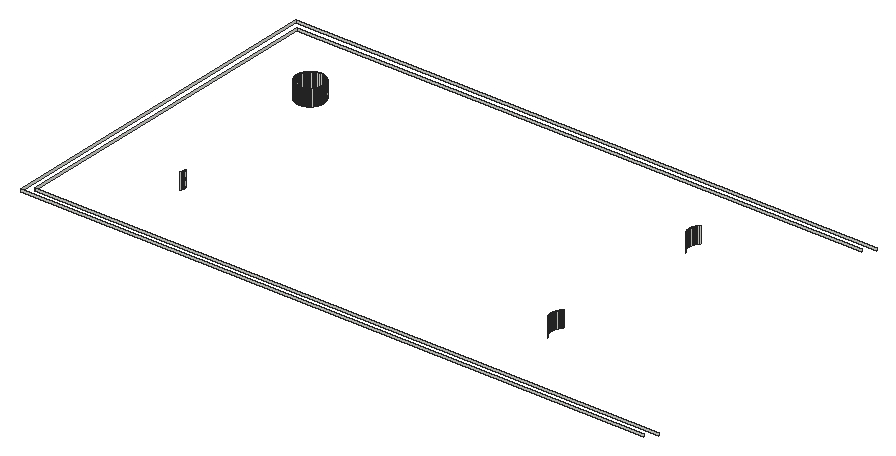
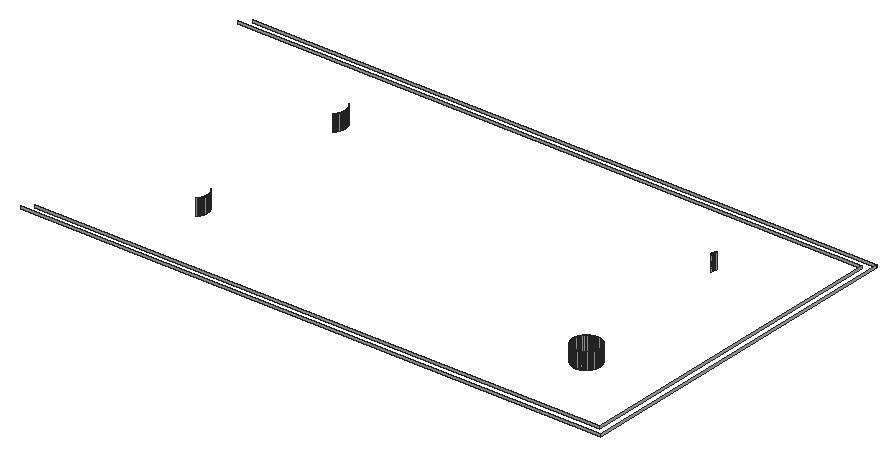
# SketchUp Ruby script. Lengths in inches.
U = 1.inch
M = Sketchup.active_model
def pt(a) = Geom::Point3d.new(a.map { |v| v * U })
def face(e, loops, mat)
  f = e.add_face(loops[0].map { |a| pt(a) })
  loops[1..].each { |l| e.add_face(l.map { |a| pt(a) }).erase! }
  f.material = f.back_material = mat if mat
  f
end
# faces: each face lists its corners as indices into pts; further lists are holes
def faces(e, pts, list, mat = nil) = list.each { |f| face(e, (f[0].is_a?(Array) ? f : [f]).map { |l| l.map { |i| pts[i] } }, mat) }
# xy, xz, yz: faces in a plane at the given z, y or x. An outline is a flat list of corners, or four numbers for a rectangle; further outlines are holes
def ring(l) = l.size == 4 ? [[l[0], l[1]], [l[2], l[1]], [l[2], l[3]], [l[0], l[3]]] : l.each_slice(2).to_a
def flat(e, list, mat, &to3) = list.each { |f| face(e, (f[0].is_a?(Array) ? f : [f]).map { |l| ring(l).map { |u, v| to3.(u, v) } }, mat) }
def xy(e, z, list, mat = nil) = flat(e, list, mat) { |x, y| [x, y, z] }
def xz(e, y, list, mat = nil) = flat(e, list, mat) { |x, z| [x, y, z] }
def yz(e, x, list, mat = nil) = flat(e, list, mat) { |y, z| [x, y, z] }
def lines(e, pts, list) = list.each { |a, b| e.add_line(pt(pts[a]), pt(pts[b])) }
# prism: a flat outline (further loops are holes) pulled along v
def prism(e, loops, v, mat = nil)
  f = face(e, loops, mat); d = Geom::Vector3d.new(v.map { |x| x * U })
  f.pushpull(f.normal.samedirection?(d) ? d.length : -d.length)
end
def box(e, o, s, mat = nil) = prism(e, [[o, [o[0] + s[0], o[1], o[2]], [o[0] + s[0], o[1] + s[1], o[2]], [o[0], o[1] + s[1], o[2]]]], [0, 0, s[2]], mat)
def at(x, y, z, deg = 0) = Geom::Transformation.translation(pt([x, y, z])) * Geom::Transformation.rotation(ORIGIN, Z_AXIS, deg.degrees)
def axes(o, x, y, z) = Geom::Transformation.new([*x, 0, *y, 0, *z, 0, *pt(o).to_a, 1])
def part(name) = M.definitions.add(name)
# library, detail: a bought-in or finely detailed component or shape, given as its bounding box
def library(name, o, s) = part(name).tap { |d| box(d.entities, o, s) }
def detail(e, o, s) = box(e.add_group.entities, o, s)
def put(e, d, t, mat = nil) = e.add_instance(d, t).tap { |i| i.material = mat if mat }
def group(e, t, mat = nil) = e.add_group.tap { |g| g.transformation = t; g.material = mat if mat }.entities
root = M.entities
xz(root,184,[[22,116,138,116.5]])
xz(root,185.5,[[23.5,116,139.5,116.5]])
xz(root,229.5,[[37.34,116,37.42,119],[37.42,116,37.5,119],[37.5,116,37.58,119],[37.58,116,37.66,119]])
xz(root,234.5,[[37.34,116,37.42,119],[37.42,116,37.5,119],[37.5,116,37.58,119],[37.58,116,37.66,119]])
xz(root,246.5,[[23.5,116,128.5,116.5]])
xz(root,248,[[22,116,130,116.5]])
yz(root,22,[[184,116,248,116.5]])
yz(root,23.5,[[185.5,116,246.5,116.5]])
yz(root,35,[[231.84,116,231.92,119],[231.92,116,232,119],[232,116,232.08,119],[232.08,116,232.16,119]])
yz(root,40,[[199.84,116,199.92,119],[199.92,116,200,119],[231.84,116,231.92,119],[231.92,116,232,119],[232,116,232.08,119],
  [232.08,116,232.16,119]])
yz(root,108,[[199.84,116,199.92,119],[199.92,116,200,119],[200,116,200.08,119],[200.08,116,200.16,119],[231.84,116,231.92,119],
  [231.92,116,232,119],[232,116,232.08,119],[232.08,116,232.16,119]])
p = [[108.73,198.23,116],[108.68,198.29,116],[108.68,198.29,119],[108.73,198.23,119],[108.79,198.18,116],[108.79,198.18,119],
  [108.625,198.35,116],[108.57,198.41,116],[108.57,198.41,119],[108.625,198.35,119],[108.52,198.47,116],[108.52,198.47,119],
  [108.48,198.53,116],[108.43,198.59,116],[108.43,198.59,119],[108.48,198.53,119],[108.39,198.66,116],[108.39,198.66,119],
  [108.35,198.73,116],[108.31,198.8,116],[108.31,198.8,119],[108.35,198.73,119],[108.27,198.87,116],[108.27,198.87,119],
  [39.79,199.01,116],[39.76,198.9375,116],[39.76,198.9375,119],[39.79,199.01,119],[108.24,198.9375,116],[108.21,199.01,116],
  [108.21,199.01,119],[108.24,198.9375,119],[39.82,199.08,116],[39.82,199.08,119],[108.18,199.08,116],[108.18,199.08,119],
  [39.85,199.15,116],[39.85,199.15,119],[108.15,199.15,116],[108.15,199.15,119],[39.88,199.23,116],[39.88,199.23,119],
  [39.9,199.3,116],[39.9,199.3,119],[108.12,199.23,116],[108.1,199.3,116],[108.1,199.3,119],[108.12,199.23,119],
  [39.92,199.38,116],[39.92,199.38,119],[108.08,199.38,116],[108.08,199.38,119],[39.94,199.45,116],[39.94,199.45,119],
  [108.06,199.45,116],[108.06,199.45,119],[39.96,199.53,116],[39.96,199.53,119],[39.97,199.61,116],[39.97,199.61,119],
  [108.04,199.53,116],[108.03,199.61,116],[108.03,199.61,119],[108.04,199.53,119],[39.98,199.6875,116],[39.98,199.6875,119],
  [108.02,199.6875,116],[108.02,199.6875,119],[39.99,199.76,116],[39.99,199.76,119],[108.01,199.76,116],[108.01,199.76,119],
  [40,199.84,116],[40,199.84,119],[108,199.84,116],[108,199.84,119],[108,200.16,116],[108.01,200.24,116],
  [108.01,200.24,119],[108,200.16,119],[108.02,200.3125,116],[108.02,200.3125,119],[108.03,200.39,116],[108.03,200.39,119],
  [108.04,200.47,116],[108.04,200.47,119],[108.06,200.55,116],[108.06,200.55,119],[108.08,200.62,116],[108.08,200.62,119],
  [108.1,200.7,116],[108.1,200.7,119],[108.12,200.77,116],[108.12,200.77,119],[108.15,200.85,116],[108.15,200.85,119],
  [108.18,200.92,116],[108.18,200.92,119],[108.21,200.99,116],[108.21,200.99,119],[108.24,201.0625,116],[108.24,201.0625,119],
  [108.27,201.13,116],[108.27,201.13,119],[108.31,201.2,116],[108.31,201.2,119],[108.35,201.27,116],[108.35,201.27,119],
  [108.39,201.34,116],[108.39,201.34,119],[108.43,201.41,116],[108.43,201.41,119],[108.48,201.47,116],[108.48,201.47,119],
  [108.52,201.53,116],[108.52,201.53,119],[108.57,201.59,116],[108.57,201.59,119],[108.625,201.65,116],[108.625,201.65,119],
  [108.68,201.71,116],[108.68,201.71,119],[108.73,201.77,116],[108.73,201.77,119],[108.79,201.82,116],[108.79,201.82,119],
  [37.03,229.54,116],[36.95,229.56,116],[36.95,229.56,119],[37.03,229.54,119],[37.11,229.53,116],[37.11,229.53,119],
  [37.1875,229.52,116],[37.1875,229.52,119],[37.26,229.51,116],[37.26,229.51,119],[37.34,229.5,116],[37.34,229.5,119],
  [37.74,229.51,116],[37.66,229.5,116],[37.66,229.5,119],[37.74,229.51,119],[37.8125,229.52,116],[37.8125,229.52,119],
  [37.89,229.53,116],[37.89,229.53,119],[37.97,229.54,116],[37.97,229.54,119],[38.05,229.56,116],[38.05,229.56,119],
  [36.65,229.65,116],[36.58,229.68,116],[36.58,229.68,119],[36.65,229.65,119],[36.73,229.62,116],[36.73,229.62,119],
  [36.8,229.6,116],[36.8,229.6,119],[36.88,229.58,116],[36.88,229.58,119],[38.12,229.58,116],[38.12,229.58,119],
  [38.2,229.6,116],[38.2,229.6,119],[38.27,229.62,116],[38.27,229.62,119],[38.35,229.65,116],[38.35,229.65,119],
  [38.42,229.68,116],[38.42,229.68,119],[36.4375,229.74,116],[36.37,229.77,116],[36.37,229.77,119],[36.4375,229.74,119],
  [36.51,229.71,116],[36.51,229.71,119],[38.49,229.71,116],[38.49,229.71,119],[38.5625,229.74,116],[38.5625,229.74,119],
  [38.63,229.77,116],[38.63,229.77,119],[36.23,229.85,116],[36.16,229.89,116],[36.16,229.89,119],[36.23,229.85,119],
  [36.3,229.81,116],[36.3,229.81,119],[38.7,229.81,116],[38.7,229.81,119],[38.77,229.85,116],[38.77,229.85,119],
  [38.84,229.89,116],[38.84,229.89,119],[36.09,229.93,116],[36.03,229.98,116],[36.03,229.98,119],[36.09,229.93,119],
  [38.91,229.93,116],[38.91,229.93,119],[38.97,229.98,116],[38.97,229.98,119],[35.97,230.02,116],[35.91,230.07,116],
  [35.91,230.07,119],[35.97,230.02,119],[39.03,230.02,116],[39.03,230.02,119],[39.09,230.07,116],[39.09,230.07,119],
  [35.85,230.125,116],[35.79,230.18,116],[35.79,230.18,119],[35.85,230.125,119],[39.15,230.125,116],[39.15,230.125,119],
  [39.21,230.18,116],[39.21,230.18,119],[35.73,230.23,116],[35.68,230.29,116],[35.68,230.29,119],[35.73,230.23,119],
  [39.27,230.23,116],[39.27,230.23,119],[39.32,230.29,116],[39.32,230.29,119],[108.73,230.23,116],[108.68,230.29,116],
  [108.68,230.29,119],[108.73,230.23,119],[108.79,230.18,116],[108.79,230.18,119],[35.625,230.35,116],[35.57,230.41,116],
  [35.57,230.41,119],[35.625,230.35,119],[39.375,230.35,116],[39.375,230.35,119],[39.43,230.41,116],[39.43,230.41,119],
  [108.625,230.35,116],[108.57,230.41,116],[108.57,230.41,119],[108.625,230.35,119],[35.52,230.47,116],[35.52,230.47,119],
  [39.48,230.47,116],[39.48,230.47,119],[108.52,230.47,116],[108.52,230.47,119],[35.48,230.53,116],[35.43,230.59,116],
  [35.43,230.59,119],[35.48,230.53,119],[39.52,230.53,116],[39.52,230.53,119],[39.57,230.59,116],[39.57,230.59,119],
  [108.48,230.53,116],[108.43,230.59,116],[108.43,230.59,119],[108.48,230.53,119],[35.39,230.66,116],[35.39,230.66,119],
  [39.61,230.66,116],[39.61,230.66,119],[108.39,230.66,116],[108.39,230.66,119],[35.35,230.73,116],[35.31,230.8,116],
  [35.31,230.8,119],[35.35,230.73,119],[39.65,230.73,116],[39.65,230.73,119],[39.69,230.8,116],[39.69,230.8,119],
  [108.35,230.73,116],[108.31,230.8,116],[108.31,230.8,119],[108.35,230.73,119],[35.27,230.87,116],[35.27,230.87,119],
  [39.73,230.87,116],[39.73,230.87,119],[108.27,230.87,116],[108.27,230.87,119],[35.24,230.9375,116],[35.21,231.01,116],
  [35.21,231.01,119],[35.24,230.9375,119],[39.76,230.9375,116],[39.76,230.9375,119],[39.79,231.01,116],[39.79,231.01,119],
  [108.24,230.9375,116],[108.21,231.01,116],[108.21,231.01,119],[108.24,230.9375,119],[35.18,231.08,116],[35.18,231.08,119],
  [39.82,231.08,116],[39.82,231.08,119],[108.18,231.08,116],[108.18,231.08,119],[35.15,231.15,116],[35.15,231.15,119],
  [39.85,231.15,116],[39.85,231.15,119],[108.15,231.15,116],[108.15,231.15,119],[35.12,231.23,116],[35.1,231.3,116],
  [35.1,231.3,119],[35.12,231.23,119],[39.88,231.23,116],[39.88,231.23,119],[39.9,231.3,116],[39.9,231.3,119],
  [108.12,231.23,116],[108.1,231.3,116],[108.1,231.3,119],[108.12,231.23,119],[35.08,231.38,116],[35.08,231.38,119],
  [39.92,231.38,116],[39.92,231.38,119],[108.08,231.38,116],[108.08,231.38,119],[35.06,231.45,116],[35.06,231.45,119],
  [39.94,231.45,116],[39.94,231.45,119],[108.06,231.45,116],[108.06,231.45,119],[35.04,231.53,116],[35.03,231.61,116],
  [35.03,231.61,119],[35.04,231.53,119],[39.96,231.53,116],[39.96,231.53,119],[39.97,231.61,116],[39.97,231.61,119],
  [108.04,231.53,116],[108.03,231.61,116],[108.03,231.61,119],[108.04,231.53,119],[35.02,231.6875,116],[35.02,231.6875,119],
  [39.98,231.6875,116],[39.98,231.6875,119],[108.02,231.6875,116],[108.02,231.6875,119],[35.01,231.76,116],[35.01,231.76,119],
  [39.99,231.76,116],[39.99,231.76,119],[108.01,231.76,116],[108.01,231.76,119],[35,231.84,116],[35,231.84,119],
  [40,231.84,116],[40,231.84,119],[108,231.84,116],[108,231.84,119],[35,232.16,116],[35.01,232.24,116],
  [35.01,232.24,119],[35,232.16,119],[35.02,232.3125,116],[35.02,232.3125,119],[39.98,232.3125,116],[39.99,232.24,116],
  [39.99,232.24,119],[39.98,232.3125,119],[40,232.16,116],[40,232.16,119],[108,232.16,116],[108.01,232.24,116],
  [108.01,232.24,119],[108,232.16,119],[108.02,232.3125,116],[108.02,232.3125,119],[35.03,232.39,116],[35.03,232.39,119],
  [39.97,232.39,116],[39.97,232.39,119],[108.03,232.39,116],[108.03,232.39,119],[35.04,232.47,116],[35.04,232.47,119],
  [39.96,232.47,116],[39.96,232.47,119],[108.04,232.47,116],[108.04,232.47,119],[35.06,232.55,116],[35.06,232.55,119],
  [35.08,232.62,116],[35.08,232.62,119],[39.92,232.62,116],[39.94,232.55,116],[39.94,232.55,119],[39.92,232.62,119],
  [108.06,232.55,116],[108.06,232.55,119],[108.08,232.62,116],[108.08,232.62,119],[35.1,232.7,116],[35.1,232.7,119],
  [39.9,232.7,116],[39.9,232.7,119],[108.1,232.7,116],[108.1,232.7,119],[35.12,232.77,116],[35.12,232.77,119],
  [39.88,232.77,116],[39.88,232.77,119],[108.12,232.77,116],[108.12,232.77,119],[35.15,232.85,116],[35.15,232.85,119],
  [35.18,232.92,116],[35.18,232.92,119],[39.82,232.92,116],[39.85,232.85,116],[39.85,232.85,119],[39.82,232.92,119],
  [108.15,232.85,116],[108.15,232.85,119],[108.18,232.92,116],[108.18,232.92,119],[35.21,232.99,116],[35.21,232.99,119],
  [39.79,232.99,116],[39.79,232.99,119],[108.21,232.99,116],[108.21,232.99,119],[35.24,233.0625,116],[35.24,233.0625,119],
  [39.76,233.0625,116],[39.76,233.0625,119],[108.24,233.0625,116],[108.24,233.0625,119],[35.27,233.13,116],[35.27,233.13,119],
  [35.31,233.2,116],[35.31,233.2,119],[39.69,233.2,116],[39.73,233.13,116],[39.73,233.13,119],[39.69,233.2,119],
  [108.27,233.13,116],[108.27,233.13,119],[108.31,233.2,116],[108.31,233.2,119],[35.35,233.27,116],[35.35,233.27,119],
  [39.65,233.27,116],[39.65,233.27,119],[108.35,233.27,116],[108.35,233.27,119],[35.39,233.34,116],[35.39,233.34,119],
  [35.43,233.41,116],[35.43,233.41,119],[39.57,233.41,116],[39.61,233.34,116],[39.61,233.34,119],[39.57,233.41,119],
  [108.39,233.34,116],[108.39,233.34,119],[108.43,233.41,116],[108.43,233.41,119],[35.48,233.47,116],[35.48,233.47,119],
  [39.52,233.47,116],[39.52,233.47,119],[108.48,233.47,116],[108.48,233.47,119],[35.52,233.53,116],[35.52,233.53,119],
  [35.57,233.59,116],[35.57,233.59,119],[39.43,233.59,116],[39.48,233.53,116],[39.48,233.53,119],[39.43,233.59,119],
  [108.52,233.53,116],[108.52,233.53,119],[108.57,233.59,116],[108.57,233.59,119],[35.625,233.65,116],[35.625,233.65,119],
  [39.375,233.65,116],[39.375,233.65,119],[108.625,233.65,116],[108.625,233.65,119],[35.68,233.71,116],[35.68,233.71,119],
  [35.73,233.77,116],[35.73,233.77,119],[39.27,233.77,116],[39.32,233.71,116],[39.32,233.71,119],[39.27,233.77,119],
  [108.68,233.71,116],[108.68,233.71,119],[108.73,233.77,116],[108.73,233.77,119],[35.79,233.82,116],[35.79,233.82,119],
  [35.85,233.875,116],[35.85,233.875,119],[39.15,233.875,116],[39.21,233.82,116],[39.21,233.82,119],[39.15,233.875,119],
  [108.79,233.82,116],[108.79,233.82,119],[35.91,233.93,116],[35.91,233.93,119],[35.97,233.98,116],[35.97,233.98,119],
  [39.03,233.98,116],[39.09,233.93,116],[39.09,233.93,119],[39.03,233.98,119],[36.03,234.02,116],[36.03,234.02,119],
  [36.09,234.07,116],[36.09,234.07,119],[38.91,234.07,116],[38.97,234.02,116],[38.97,234.02,119],[38.91,234.07,119],
  [36.16,234.11,116],[36.16,234.11,119],[36.23,234.15,116],[36.23,234.15,119],[38.77,234.15,116],[38.84,234.11,116],
  [38.84,234.11,119],[38.77,234.15,119],[36.3,234.19,116],[36.3,234.19,119],[36.37,234.23,116],[36.37,234.23,119],
  [36.4375,234.26,116],[36.4375,234.26,119],[38.5625,234.26,116],[38.63,234.23,116],[38.63,234.23,119],[38.5625,234.26,119],
  [38.7,234.19,116],[38.7,234.19,119],[36.51,234.29,116],[36.51,234.29,119],[36.58,234.32,116],[36.58,234.32,119],
  [36.65,234.35,116],[36.65,234.35,119],[38.35,234.35,116],[38.42,234.32,116],[38.42,234.32,119],[38.35,234.35,119],
  [38.49,234.29,116],[38.49,234.29,119],[36.73,234.38,116],[36.73,234.38,119],[36.8,234.4,116],[36.8,234.4,119],
  [36.88,234.42,116],[36.88,234.42,119],[36.95,234.44,116],[36.95,234.44,119],[37.03,234.46,116],[37.03,234.46,119],
  [37.97,234.46,116],[38.05,234.44,116],[38.05,234.44,119],[37.97,234.46,119],[38.12,234.42,116],[38.12,234.42,119],
  [38.2,234.4,116],[38.2,234.4,119],[38.27,234.38,116],[38.27,234.38,119],[37.11,234.47,116],[37.11,234.47,119],
  [37.1875,234.48,116],[37.1875,234.48,119],[37.26,234.49,116],[37.26,234.49,119],[37.34,234.5,116],[37.34,234.5,119],
  [37.66,234.5,116],[37.74,234.49,116],[37.74,234.49,119],[37.66,234.5,119],[37.8125,234.48,116],[37.8125,234.48,119],
  [37.89,234.47,116],[37.89,234.47,119]]
faces(root,p,[[0,1,2,3],[4,0,3,5],[6,7,8,9],[1,6,9,2],[7,10,11,8],[12,13,14,15],[10,12,15,11],[13,16,17,14],
  [18,19,20,21],[16,18,21,17],[19,22,23,20],[24,25,26,27],[28,29,30,31],[22,28,31,23],[32,24,27,33],[29,34,35,30],
  [36,32,33,37],[34,38,39,35],[40,36,37,41],[42,40,41,43],[44,45,46,47],[38,44,47,39],[48,42,43,49],[45,50,51,46],
  [52,48,49,53],[50,54,55,51],[56,52,53,57],[58,56,57,59],[60,61,62,63],[54,60,63,55],[64,58,59,65],[61,66,67,62],
  [68,64,65,69],[66,70,71,67],[72,68,69,73],[70,74,75,71],[76,77,78,79],[77,80,81,78],[80,82,83,81],[82,84,85,83],
  [84,86,87,85],[86,88,89,87],[88,90,91,89],[90,92,93,91],[92,94,95,93],[94,96,97,95],[96,98,99,97],[98,100,101,99],
  [100,102,103,101],[102,104,105,103],[104,106,107,105],[106,108,109,107],[108,110,111,109],[110,112,113,111],[112,114,115,113],[114,116,117,115],
  [116,118,119,117],[118,120,121,119],[120,122,123,121],[122,124,125,123],[126,127,128,129],[130,126,129,131],[132,130,131,133],[134,132,133,135],
  [136,134,135,137],[138,139,140,141],[142,138,141,143],[144,142,143,145],[146,144,145,147],[148,146,147,149],[150,151,152,153],[154,150,153,155],
  [156,154,155,157],[158,156,157,159],[127,158,159,128],[160,148,149,161],[162,160,161,163],[164,162,163,165],[166,164,165,167],[168,166,167,169],
  [170,171,172,173],[174,170,173,175],[151,174,175,152],[176,168,169,177],[178,176,177,179],[180,178,179,181],[182,183,184,185],[186,182,185,187],
  [171,186,187,172],[188,180,181,189],[190,188,189,191],[192,190,191,193],[194,195,196,197],[183,194,197,184],[198,192,193,199],[200,198,199,201],
  [202,203,204,205],[195,202,205,196],[206,200,201,207],[208,206,207,209],[210,211,212,213],[203,210,213,204],[214,208,209,215],[216,214,215,217],
  [218,219,220,221],[211,218,221,212],[222,216,217,223],[224,222,223,225],[226,227,228,229],[230,226,229,231],[232,233,234,235],[219,232,235,220],
  [236,224,225,237],[238,236,237,239],[240,241,242,243],[227,240,243,228],[233,244,245,234],[246,238,239,247],[241,248,249,242],[250,251,252,253],
  [244,250,253,245],[254,246,247,255],[256,254,255,257],[258,259,260,261],[248,258,261,249],[251,262,263,252],[264,256,257,265],[259,266,267,260],
  [268,269,270,271],[262,268,271,263],[272,264,265,273],[274,272,273,275],[276,277,278,279],[266,276,279,267],[269,280,281,270],[282,274,275,283],
  [277,284,285,278],[286,287,288,289],[280,286,289,281],[290,282,283,291],[292,290,291,293],[294,295,296,297],[284,294,297,285],[287,298,299,288],
  [300,292,293,301],[295,302,303,296],[298,304,305,299],[306,300,301,307],[302,308,309,303],[310,311,312,313],[304,310,313,305],[314,306,307,315],
  [316,314,315,317],[318,319,320,321],[308,318,321,309],[311,322,323,312],[324,316,317,325],[319,326,327,320],[322,328,329,323],[330,324,325,331],
  [326,332,333,327],[334,335,336,337],[328,334,337,329],[338,330,331,339],[340,338,339,341],[342,343,344,345],[332,342,345,333],[335,346,347,336],
  [348,340,341,349],[343,350,351,344],[346,352,353,347],[354,348,349,355],[350,356,357,351],[352,358,359,353],[360,354,355,361],[356,362,363,357],
  [364,365,366,367],[365,368,369,366],[370,371,372,373],[371,374,375,372],[376,377,378,379],[377,380,381,378],[368,382,383,369],[384,370,373,385],
  [380,386,387,381],[382,388,389,383],[390,384,385,391],[386,392,393,387],[388,394,395,389],[394,396,397,395],[398,399,400,401],[399,390,391,400],
  [392,402,403,393],[402,404,405,403],[396,406,407,397],[408,398,401,409],[404,410,411,405],[406,412,413,407],[414,408,409,415],[410,416,417,411],
  [412,418,419,413],[418,420,421,419],[422,423,424,425],[423,414,415,424],[416,426,427,417],[426,428,429,427],[420,430,431,421],[432,422,425,433],
  [428,434,435,429],[430,436,437,431],[438,432,433,439],[434,440,441,435],[436,442,443,437],[442,444,445,443],[446,447,448,449],[447,438,439,448],
  [440,450,451,441],[450,452,453,451],[444,454,455,445],[456,446,449,457],[452,458,459,453],[454,460,461,455],[460,462,463,461],[464,465,466,467],
  [465,456,457,466],[458,468,469,459],[468,470,471,469],[462,472,473,463],[474,464,467,475],[470,476,477,471],[472,478,479,473],[478,480,481,479],
  [482,483,484,485],[483,474,475,484],[476,486,487,477],[486,488,489,487],[480,490,491,481],[492,482,485,493],[488,494,495,489],[490,496,497,491],
  [496,498,499,497],[500,501,502,503],[501,492,493,502],[494,504,505,495],[504,506,507,505],[498,508,509,499],[508,510,511,509],[512,513,514,515],
  [513,500,503,514],[506,516,517,507],[510,518,519,511],[518,520,521,519],[522,523,524,525],[523,512,515,524],[520,526,527,521],[526,528,529,527],
  [530,531,532,533],[531,522,525,532],[528,534,535,529],[534,536,537,535],[538,539,540,541],[539,530,533,540],[536,542,543,537],[542,544,545,543],
  [544,546,547,545],[548,549,550,551],[549,552,553,550],[552,538,541,553],[546,554,555,547],[554,556,557,555],[556,558,559,557],[560,561,562,563],
  [561,564,565,562],[564,548,551,565],[558,566,567,559],[566,568,569,567],[568,570,571,569],[570,572,573,571],[572,574,575,573],[576,577,578,579],
  [577,580,581,578],[580,582,583,581],[582,584,585,583],[584,560,563,585],[574,586,587,575],[586,588,589,587],[588,590,591,589],[590,592,593,591],
  [594,595,596,597],[595,598,599,596],[598,600,601,599],[600,576,579,601]])
